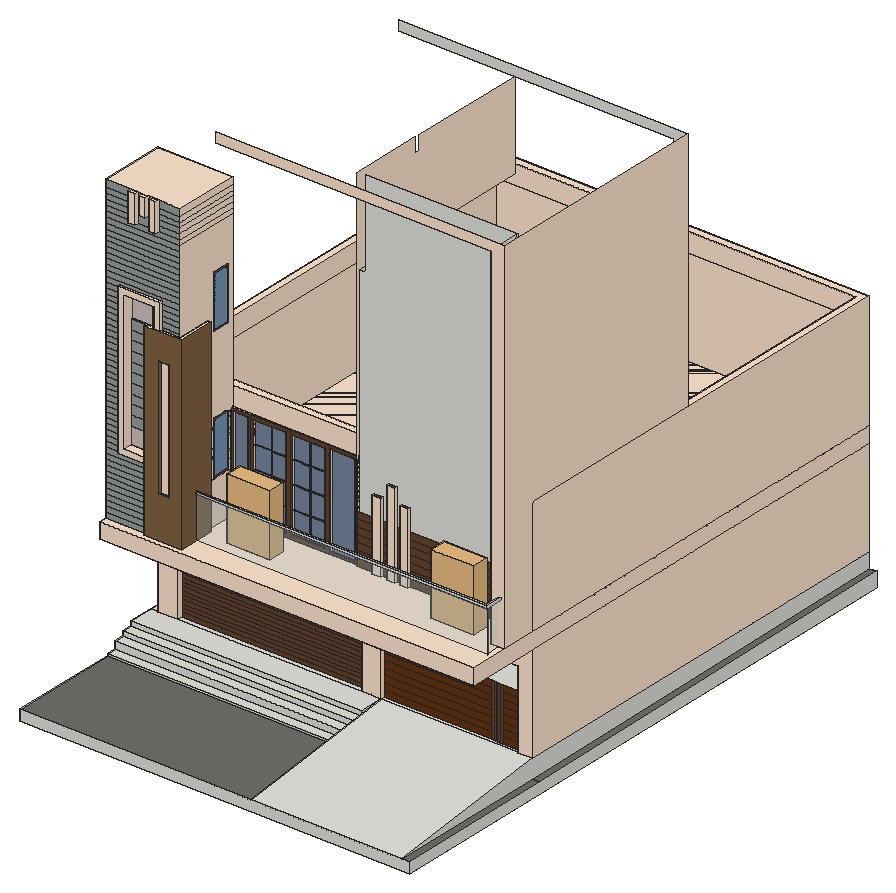
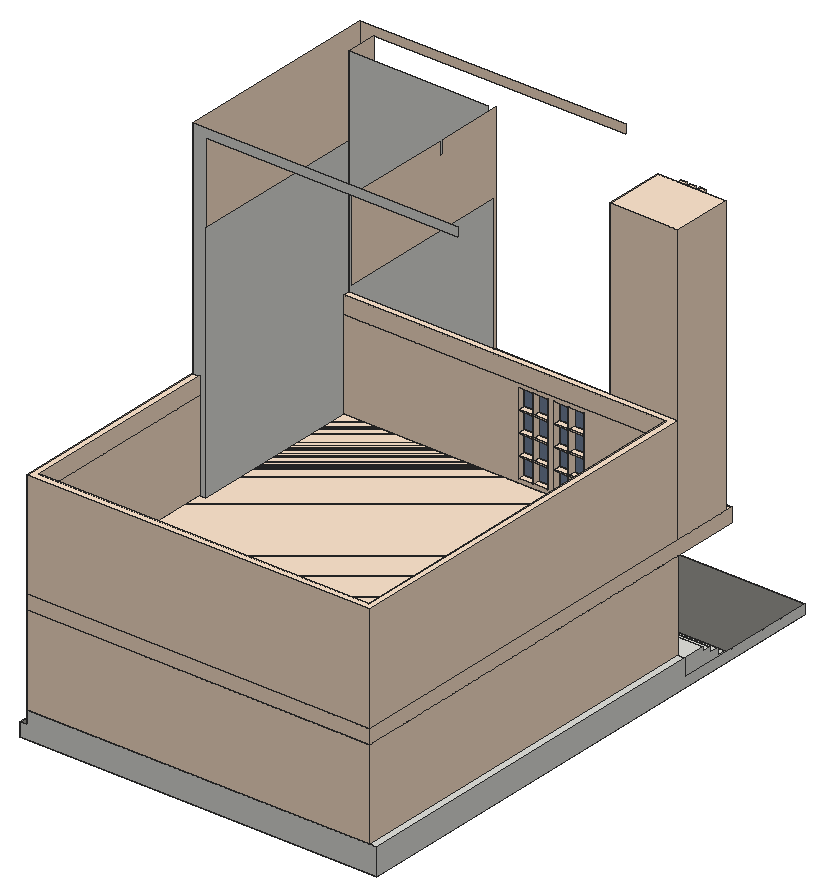
# SketchUp Ruby script. Lengths in inches.
U = 1.inch
M = Sketchup.active_model
def pt(a) = Geom::Point3d.new(a.map { |v| v * U })
def face(e, loops, mat)
  f = e.add_face(loops[0].map { |a| pt(a) })
  loops[1..].each { |l| e.add_face(l.map { |a| pt(a) }).erase! }
  f.material = f.back_material = mat if mat
  f
end
# faces: each face lists its corners as indices into pts; further lists are holes
def faces(e, pts, list, mat = nil) = list.each { |f| face(e, (f[0].is_a?(Array) ? f : [f]).map { |l| l.map { |i| pts[i] } }, mat) }
# xy, xz, yz: faces in a plane at the given z, y or x. An outline is a flat list of corners, or four numbers for a rectangle; further outlines are holes
def ring(l) = l.size == 4 ? [[l[0], l[1]], [l[2], l[1]], [l[2], l[3]], [l[0], l[3]]] : l.each_slice(2).to_a
def flat(e, list, mat, &to3) = list.each { |f| face(e, (f[0].is_a?(Array) ? f : [f]).map { |l| ring(l).map { |u, v| to3.(u, v) } }, mat) }
def xy(e, z, list, mat = nil) = flat(e, list, mat) { |x, y| [x, y, z] }
def xz(e, y, list, mat = nil) = flat(e, list, mat) { |x, z| [x, y, z] }
def yz(e, x, list, mat = nil) = flat(e, list, mat) { |y, z| [x, y, z] }
def lines(e, pts, list) = list.each { |a, b| e.add_line(pt(pts[a]), pt(pts[b])) }
# prism: a flat outline (further loops are holes) pulled along v
def prism(e, loops, v, mat = nil)
  f = face(e, loops, mat); d = Geom::Vector3d.new(v.map { |x| x * U })
  f.pushpull(f.normal.samedirection?(d) ? d.length : -d.length)
end
def box(e, o, s, mat = nil) = prism(e, [[o, [o[0] + s[0], o[1], o[2]], [o[0] + s[0], o[1] + s[1], o[2]], [o[0], o[1] + s[1], o[2]]]], [0, 0, s[2]], mat)
def at(x, y, z, deg = 0) = Geom::Transformation.translation(pt([x, y, z])) * Geom::Transformation.rotation(ORIGIN, Z_AXIS, deg.degrees)
def axes(o, x, y, z) = Geom::Transformation.new([*x, 0, *y, 0, *z, 0, *pt(o).to_a, 1])
def part(name) = M.definitions.add(name)
# library, detail: a bought-in or finely detailed component or shape, given as its bounding box
def library(name, o, s) = part(name).tap { |d| box(d.entities, o, s) }
def detail(e, o, s) = box(e.add_group.entities, o, s)
def put(e, d, t, mat = nil) = e.add_instance(d, t).tap { |i| i.material = mat if mat }
def group(e, t, mat = nil) = e.add_group.tap { |g| g.transformation = t; g.material = mat if mat }.entities
root = M.entities
M.materials.add("C01_Vanilla_Cream").color = [255, 230, 206]
M.materials.add("Glass_Mirror_01").color = [119, 135, 160]
M.materials.add("Glass_Mirror_2").color = [118, 153, 185]
M.materials.add("Glass_Safety_1").color = [204, 235, 244]
M.materials["Glass_Safety_1"].alpha = 0.25
M.materials.add("Glass_Sky Reflection_01").color = [126, 138, 183]
M.materials["Glass_Sky Reflection_01"].alpha = 0.25
M.materials.add("M03_Pewter_Shine").color = [152, 160, 157]
M.materials.add("Plywood_01_1K").color = [104, 52, 18]
M.materials.add("Plywood_01_1K1").color = [130, 99, 66]
M.materials.add("Plywood_01_1K2").color = [125, 96, 64]
M.materials.add("Tile_Exterior_07_1K").color = [112, 111, 107]
M.materials.add("Wood_Veneer_15_1K").color = [103, 69, 45]
c1 = library("Group_2",[-1.28,-0.39,0],[21.22,20.51,48.44])
xy(root,139,[[465.23,139.58,463.25,158.82,463.38,158.82,465.57,139.58],[453,158.82,453,441,471,441,471,158.82,463.38,158.82,462,170.99,462,158.82],[462,158.82,462,170.99,463.25,158.82],[463.25,158.82,462,170.99,463.38,158.82],[278.18,194.51,288.54,198],
  [256.9,198,453,201]])
xy(root,191.09,[[105.48,138.27,465.23,139.58],[105.48,139.58,105.48,141.07,462.4,141.07,462.4,165.41,462.58,165.41,465.23,139.58],[465.23,139.58,462.58,165.41,465.23,165.41]])
xz(root,138.27,[[105.48,191.09,465.23,193.67]])
xz(root,139.58,[[465.23,139,465.57,191.09],[105.48,191.09,465.57,191.09,462,191.2,105.48,191.2]])
xz(root,139.58,[[105.48,139,465.23,191.09]],"Glass_Safety_1")
xz(root,141.07,[[105.48,191.09,462.4,193.67]])
xz(root,158.82,[[453,139,471,139,471,585,114,585,114,573,453,573]],"C01_Vanilla_Cream")
xz(root,165.41,[[462.4,191.09,465.23,193.67]])
xz(root,194.51,[[278.18,139,288.54,225.8],[296.18,139,306.54,243.16],[312.12,139,322.48,225.8]],"C01_Vanilla_Cream")
xz(root,198,[[256.9,139,278.18,147.68],[278.18,139,288.54,147.68],[288.54,139,296.18,147.68],[296.18,139,306.54,147.68],[306.54,139,312.12,147.68],
  [312.12,139,322.48,147.68],[322.48,139,453,147.68],[256.9,147.68,278.18,156.36],[278.18,147.68,288.54,225.8],[288.54,147.68,296.18,156.36],
  [296.18,147.68,306.54,243.16],[306.54,147.68,312.12,156.36],[312.12,147.68,322.48,225.8],[322.48,147.68,453,156.36],[256.9,156.36,278.18,165.04],
  [288.54,156.36,296.18,165.04],[306.54,156.36,312.12,165.04],[322.48,156.36,453,165.04],[256.9,165.04,278.18,173.72],[288.54,165.04,296.18,173.72],
  [306.54,165.04,312.12,173.72],[322.48,165.04,453,173.72],[256.9,173.72,278.18,182.4],[288.54,173.72,296.18,182.4],[306.54,173.72,312.12,182.4],
  [322.48,173.72,453,182.4],[256.9,182.4,278.18,191.08],[288.54,182.4,296.18,191.08],[306.54,182.4,312.12,191.08],[322.48,182.4,453,191.08],
  [256.9,191.08,278.18,199.76],[288.54,191.08,296.18,199.76],[306.54,191.08,312.12,199.76],[322.48,191.08,453,199.76]],"Wood_Veneer_15_1K")
xz(root,201,[[256.9,139,256.9,465,265.5,465,265.5,573,453,573,453,139]])
xz(root,205.5,[[284.33,0,416.71,8.16],[430.63,0,453,8.16],[284.33,8.16,416.71,16.33],[430.63,8.16,453,16.33],[284.33,16.33,416.71,24.49],
  [430.63,16.33,453,24.49],[284.33,24.49,416.71,32.65],[430.63,24.49,453,32.65],[284.33,32.65,416.71,40.82],[430.63,32.65,453,40.82],
  [284.33,40.82,416.71,48.98],[430.63,40.82,453,48.98],[284.33,48.98,416.71,57.14],[430.63,48.98,453,57.14],[284.33,57.14,416.71,65.31],
  [430.63,57.14,453,65.31]],"Plywood_01_1K")
xz(root,205.5,[[416.71,0,419.71,65.31],[419.71,0,422.27,65.31],[422.27,0,425.27,65.31],[425.27,0,427.63,65.31],[427.63,0,430.63,65.31]],"Wood_Veneer_15_1K")
xz(root,441,[[453,139,453,573,114,573,114,585,471,585,471,139]])
yz(root,105.48,[[138.27,191.09,141.07,193.67]])
yz(root,256.9,[[198,139,198,573,287.91,573,287.91,555.9375,293.09,555.9375,293.09,573,441,573,441,465,201,465,201,139]],"C01_Vanilla_Cream")
yz(root,278.18,[[194.51,139,198,225.8]],"C01_Vanilla_Cream")
yz(root,288.54,[[194.51,139,198,225.8]],"C01_Vanilla_Cream")
yz(root,296.18,[[194.51,139,198,243.16]],"C01_Vanilla_Cream")
yz(root,306.54,[[194.51,139,198,243.16]],"C01_Vanilla_Cream")
yz(root,312.12,[[194.51,139,198,225.8]])
yz(root,322.48,[[194.51,139,198,225.8]],"C01_Vanilla_Cream")
yz(root,453,[[198,139,201,573],[201,139,441,465]])
yz(root,453,[[158.82,139,198,573]],"C01_Vanilla_Cream")
yz(root,462.4,[[141.07,191.09,165.41,193.67]])
yz(root,465.23,[[138.27,191.09,165.41,193.67]])
yz(root,471,[[158.82,139,441,585]],"C01_Vanilla_Cream")
p = [[465.23,139.58,191.09],[462.58,165.41,191.09],[462,170.99,191.09],[462,170.99,139],[463.25,158.82,139],[465.23,139.58,139],
  [105.48,139.58,191.2],[105.48,139.58,193],[2323.11,2299.07,-227.3],[2323.11,2299.07,-224.27],[2323.11,2299.07,-230.33],[2331.43,2299.07,-221.25],
  [2331.45,2299.07,-233.35],[2331.43,2299.07,-233.35],[2331.45,2299.07,-221.25]]
faces(root,p,[[0,1,2,3,4,5]],"Glass_Safety_1")
lines(root,p,[[6,7],[8,9],[10,8],[9,11],[12,13],[11,14],[13,10]])
g1 = group(root,at(0,0,-36))
xy(g1,0,[[0,0,480,720]])
xy(g1,12.99,[[284.33,0,471,201]])
xy(g1,12.99,[[0,0,284.33,134.43],[471,0,480,201]],"Tile_Exterior_07_1K")
xy(g1,15.375,[[0,134.43,284.33,146.43]])
xy(g1,24.09,[[0,146.43,284.33,158.43]])
xy(g1,30.22,[[0,158.43,284.33,170.43]])
xy(g1,36,[[0,170.43,284.33,201],[0,201,471,720]])
xz(g1,0,[[0,0,480,12.99]])
xz(g1,134.43,[[0,12.99,284.33,15.375]])
xz(g1,146.43,[[0,15.375,284.33,24.09]])
xz(g1,158.43,[[0,24.09,284.33,30.22]])
xz(g1,170.43,[[0,30.22,284.33,36]])
xz(g1,720,[[0,0,0,36,471,36,471,18,480,18,480,0]])
yz(g1,0,[[0,0,0,12.99,201,12.99,201,36,720,36,720,0],[134.43,12.99,134.43,15.375,146.43,15.375,146.43,24.09,158.43,24.09,158.43,30.22,170.43,30.22,170.43,36,201,36,201,12.99]])
yz(g1,284.33,[[0,12.99,170.43,32.5,170.43,30.22,158.43,30.22,158.43,24.09,146.43,24.09,146.43,15.375,134.43,15.375,134.43,12.99],[134.43,12.99,201,12.99,201,36,170.43,32.5,170.43,30.22,158.43,30.22,158.43,24.09,146.43,24.09,146.43,15.375,134.43,15.375],[170.43,32.5,201,36,170.43,36]])
yz(g1,471,[[0,12.99,201,12.99,720,18,720,36,201,36]])
yz(g1,480,[[0,0,720,0,720,18,201,12.99,0,12.99]])
p = [[284.33,201,36],[284.33,170.43,32.5],[284.33,0,12.99],[457.43,0,12.99],[471,0,12.99],[471,201,36],
  [480,201,12.99],[480,720,18],[471,720,18],[471,201,12.99]]
faces(g1,p,[[0,1,2,3,4,5]])
faces(g1,p,[[6,7,8,9]],"Tile_Exterior_07_1K")
g2 = group(root,at(9,201,0),"C01_Vanilla_Cream")
xy(g2,0,[[[0,0,24,0,24,6.24,251.33,6.24,251.33,0,263.33,0,275.33,9,275.33,188.59,453,188.59,453,9,444,9,444,0,462,0,462,519,0,519],[9,9,9,510,453,510,453,200.35,263.33,200.35,263.33,9]],[263.33,0,275.33,0,275.33,9],[9,9,263.33,9,263.33,200.35,453,200.35,453,510,9,510],[275.33,9,453,188.59]])
xy(g2,7.84,[[327.57,194.47,371.57,200.35]])
xy(g2,7.84,[[327.57,188.59,371.57,194.47]],"Wood_Veneer_15_1K")
xy(g2,96,[[24,0,251.33,6.24],[275.33,0,444,9]])
xy(g2,100.92,[[327.57,194.47,371.57,200.35]])
xy(g2,100.92,[[327.57,188.59,371.57,194.47]],"Wood_Veneer_15_1K")
xy(g2,120,[[[0,0,462,519],[9,9,9,510,453,510,453,200.35,263.33,200.35,263.33,9],[275.33,9,453,188.59]]])
xz(g2,0,[[0,0,24,0,24,96,251.33,96,251.33,0,275.33,0,275.33,96,444,96,444,0,462,0,462,120,0,120]])
xz(g2,6.24,[[24,0,251.33,4.8],[24,4.8,251.33,9.6],[24,9.6,251.33,14.4],[24,14.4,251.33,19.2],[24,19.2,251.33,24],
  [24,24,251.33,28.8],[24,28.8,251.33,33.6],[24,33.6,251.33,38.4],[24,38.4,251.33,43.2],[24,43.2,251.33,48],
  [24,48,251.33,52.8],[24,52.8,251.33,57.6],[24,57.6,251.33,62.4],[24,62.4,251.33,67.2],[24,67.2,251.33,72],
  [24,72,251.33,76.8],[24,76.8,251.33,81.6],[24,81.6,251.33,86.4],[24,86.4,251.33,91.2],[24,91.2,251.33,96]],"Wood_Veneer_15_1K")
xz(g2,9,[[9,0,263.33,120],[444,0,444,96,275.33,96,275.33,120,453,120,453,0]])
xz(g2,188.59,[[[275.33,0,453,120],[327.57,7.84,371.57,100.92]]],"Plywood_01_1K2")
xz(g2,194.47,[[327.57,7.84,371.57,100.92]],"Wood_Veneer_15_1K")
xz(g2,200.35,[[[263.33,0,453,120],[327.57,7.84,371.57,100.92]]])
xz(g2,510,[[9,0,453,120]])
xz(g2,519,[[0,0,462,120]])
yz(g2,0,[[0,0,519,120]])
yz(g2,9,[[9,0,510,120]])
yz(g2,24,[[0,0,6.24,96]])
yz(g2,251.33,[[0,0,6.24,96]])
yz(g2,263.33,[[9,0,200.35,120]])
yz(g2,275.33,[[0,0,188.59,0,188.59,120,9,120,9,96,0,96]])
yz(g2,327.57,[[194.47,7.84,200.35,100.92]])
yz(g2,327.57,[[188.59,7.84,194.47,100.92]],"Wood_Veneer_15_1K")
yz(g2,371.57,[[194.47,7.84,200.35,100.92]])
yz(g2,371.57,[[188.59,7.84,194.47,100.92]],"Wood_Veneer_15_1K")
yz(g2,444,[[0,0,9,96]])
yz(g2,453,[[9,0,188.59,120],[188.59,0,200.35,120],[200.35,0,510,120]])
yz(g2,462,[[0,0,519,120]])
p = [[263.33,0,0],[263.33,9,120]]
lines(g2,p,[[0,1]])
g3 = group(root,at(9,201,120),"C01_Vanilla_Cream")
xy(g3,0,[[0,-89.98,462,519]])
xy(g3,19,[[0,-89.98,462,-89.98,462,519,0,519,0,0,91.9,0,91.9,-38.7,96.48,-38.7,96.48,-84.13,50.47,-84.13,50.47,-80.45,0,-80.45],[0,-80.45,91.9,0]])
xy(g3,71.29,[[68.81,-84.13,81.2,-81.02]],"Plywood_01_1K1")
xy(g3,97.51,[[17.03,-83.45,50.47,-80.45]])
xy(g3,104.51,[[24.03,-83.45,50.47,-83.45,50.47,-80.45,61.96,-80.45,61.96,-71.76,24.03,-71.76]])
xy(g3,217.73,[[68.81,-84.13,81.2,-81.02]],"Plywood_01_1K1")
xy(g3,243.18,[[24.03,-71.76,50.48,-69.76]])
xy(g3,250.46,[[50.47,-84.13,96.48,-84.13,96.48,-38.7,91.9,-38.7,91.9,-80.45,50.47,-80.45]])
xy(g3,250.6,[[61.96,-83.45,68.96,-80.45]])
xy(g3,275.37,[[24.03,-83.45,24.03,-69.76,50.48,-69.76,50.48,-71.76,61.96,-71.76,61.96,-83.45]])
xy(g3,282.37,[[17.03,-83.45,68.96,-80.45]])
xy(g3,358.04,[[31.4,-85.45,39.37,-80.45],[57.05,-85.45,65.02,-80.45]])
xy(g3,371.08,[[44.54,-85.45,52.51,-80.45]])
xy(g3,393,[[31.4,-85.45,39.37,-80.45],[44.54,-85.45,52.51,-80.45],[57.05,-85.45,65.02,-80.45],[0,-80.45,91.9,0]])
xz(g3,-89.98,[[0,0,462,19]])
xz(g3,-85.45,[[31.4,358.04,39.37,393],[57.05,358.04,65.02,393],[44.54,371.08,52.51,393]])
xz(g3,-84.13,[[[50.47,19,96.48,250.46],[68.81,71.29,81.2,217.73]]],"Plywood_01_1K1")
xz(g3,-83.45,[[17.03,97.51,50.47,97.51,50.47,104.51,24.03,104.51,24.03,275.37,61.96,275.37,61.96,250.6,68.96,250.6,68.96,282.37,17.03,282.37]])
xz(g3,-81.02,[[68.81,71.29,81.2,217.73]])
xz(g3,-80.45,[[50.47,19,91.9,25.52],[50.47,25.52,91.9,32.04],[50.47,32.04,91.9,38.56],[50.47,38.56,91.9,45.08],[50.47,45.08,91.9,51.6],
  [50.47,51.6,91.9,58.12],[50.47,58.12,91.9,64.64],[50.47,64.64,91.9,64.64,91.9,247.2,68.96,247.2,68.96,250.46,61.96,250.46,61.96,104.51,50.47,104.51],[50.47,104.51,61.96,250.46],[61.96,250.46,68.96,250.6],
  [31.4,358.04,39.37,393],[57.05,358.04,65.02,393],[44.54,371.08,52.51,393]])
xz(g3,-80.45,[[0,19,50.47,25.52],[0,25.52,50.47,32.04],[0,32.04,50.47,38.56],[0,38.56,50.47,45.08],[0,45.08,50.47,51.6],
  [0,51.6,50.47,58.12],[0,58.12,50.47,64.64],[0,64.64,50.47,71.16],[0,71.16,50.47,77.68],[0,77.68,50.47,84.2],
  [0,84.2,50.47,90.72],[0,90.72,50.47,97.24],[0,97.24,50.47,97.24,50.47,97.51,17.03,97.51,17.03,103.76,0,103.76],[0,103.76,17.03,110.28],[0,110.28,17.03,116.8],
  [0,116.8,17.03,123.32],[0,123.32,17.03,129.84],[0,129.84,17.03,136.36],[0,136.36,17.03,142.88],[0,142.88,17.03,149.4],
  [0,149.4,17.03,155.92],[0,155.92,17.03,162.44],[0,162.44,17.03,168.96],[0,168.96,17.03,175.48],[0,175.48,17.03,182],
  [0,182,17.03,188.52],[0,188.52,17.03,195.04],[0,195.04,17.03,201.56],[0,201.56,17.03,208.08],[0,208.08,17.03,214.6],
  [0,214.6,17.03,221.12],[0,221.12,17.03,227.64],[0,227.64,17.03,234.16],[0,234.16,17.03,240.68],[0,240.68,17.03,247.2],
  [0,247.2,17.03,253.72],[68.96,247.2,91.9,250.46],[68.96,250.46,91.9,253.72],[0,253.72,17.03,260.24],[68.96,253.72,91.9,260.24],
  [0,260.24,17.03,266.76],[68.96,260.24,91.9,266.76],[0,266.76,17.03,273.28],[68.96,266.76,91.9,273.28],[0,273.28,17.03,279.8],
  [68.96,273.28,91.9,279.8],[0,279.8,17.03,279.8,17.03,282.37,68.96,282.37,68.96,279.8,91.9,279.8,91.9,286.32,0,286.32],[0,286.32,91.9,292.84],[0,292.84,91.9,299.36],[0,299.36,91.9,305.88],
  [0,305.88,91.9,312.4],[0,312.4,91.9,318.92],[0,318.92,91.9,325.44],[0,325.44,91.9,331.96],[0,331.96,91.9,338.48],
  [0,338.48,91.9,345],[0,345,91.9,351.52],[0,351.52,91.9,358.04],[0,358.04,31.4,364.56],[39.37,358.04,57.05,358.04,57.05,393,52.51,393,52.51,371.08,44.54,371.08,44.54,393,39.37,393],
  [65.02,358.04,91.9,364.56],[0,364.56,31.4,371.08],[65.02,364.56,91.9,371.08],[0,371.08,31.4,377.6],[65.02,371.08,91.9,377.6],
  [0,377.6,31.4,384.12],[65.02,377.6,91.9,384.12],[0,384.12,31.4,393],[65.02,384.12,91.9,393]],"M03_Pewter_Shine")
xz(g3,-71.76,[[24.03,104.51,61.96,125.46]],"Glass_Sky Reflection_01")
xz(g3,-71.76,[[24.03,125.46,61.96,137.23],[24.03,137.23,61.96,149.01],[24.03,149.01,61.96,160.78],[24.03,160.78,61.96,172.55],[24.03,172.55,61.96,184.32],
  [24.03,184.32,61.96,196.09],[24.03,196.09,61.96,207.87],[24.03,207.87,61.96,219.64],[24.03,219.64,61.96,231.41],[24.03,231.41,61.96,243.18],
  [50.48,243.18,61.96,249.62],[50.48,249.62,61.96,256.06],[50.48,256.06,61.96,262.5],[50.48,262.5,61.96,268.93],[50.48,268.93,61.96,275.37]],"M03_Pewter_Shine")
xz(g3,-69.76,[[24.03,243.18,50.48,275.37]],"Glass_Sky Reflection_01")
xz(g3,-38.7,[[91.9,19,96.48,250.46]])
xz(g3,0,[[0,19,91.9,393]])
xz(g3,519,[[0,0,462,19]])
yz(g3,0,[[-89.98,0,519,19],[-80.45,19,0,393]])
yz(g3,17.03,[[-83.45,97.51,-80.45,282.37]])
yz(g3,24.03,[[-83.45,104.51,-71.76,104.51,-71.76,243.18,-69.76,243.18,-69.76,275.37,-83.45,275.37]])
yz(g3,31.4,[[-85.45,358.04,-80.45,393]])
yz(g3,39.37,[[-85.45,358.04,-80.45,393]])
yz(g3,44.54,[[-85.45,371.08,-80.45,393]])
yz(g3,50.47,[[-84.13,19,-84.13,250.46,-83.45,250.46,-83.45,97.51,-80.45,97.51,-80.45,19],[-83.45,97.51,-80.45,104.51],[-83.45,104.51,-80.45,250.46]])
yz(g3,50.48,[[-71.76,243.18,-69.76,249.62],[-71.76,249.62,-69.76,256.06],[-71.76,256.06,-69.76,262.5],[-71.76,262.5,-69.76,268.93],[-71.76,268.93,-69.76,275.37]])
yz(g3,52.51,[[-85.45,371.08,-80.45,393]])
yz(g3,57.05,[[-85.45,358.04,-80.45,393]])
yz(g3,61.96,[[-80.45,104.51,-80.45,250.6,-83.45,250.6,-83.45,275.37,-71.76,275.37,-71.76,104.51]])
yz(g3,65.02,[[-85.45,358.04,-80.45,393]])
yz(g3,68.81,[[-84.13,71.29,-81.02,217.73]],"Plywood_01_1K1")
yz(g3,68.96,[[-83.45,250.6,-80.45,282.37]])
yz(g3,81.2,[[-84.13,71.29,-81.02,217.73]],"Plywood_01_1K1")
yz(g3,91.9,[[-80.45,19,-38.7,250.46],[[-38.7,19,0,19,0,351.52,-80.45,351.52,-80.45,250.46,-38.7,250.46],[-30.47,71.51,-5.73,139.15],[-30.47,233.3,-5.73,300.9375]],[-80.45,351.52,0,358.04],[-80.45,358.04,0,364.56],[-80.45,364.56,0,371.08],
  [-80.45,371.08,0,377.6],[-80.45,377.6,0,384.12],[-80.45,384.12,0,393]])
yz(g3,91.9,[[-27.47,74.51,-8.73,136.15],[-27.47,236.3,-8.73,297.9375]],"Glass_Mirror_2")
yz(g3,91.9,[[[-30.47,71.51,-5.73,139.15],[-27.47,74.51,-8.73,136.15]],[[-30.47,233.3,-5.73,300.9375],[-27.47,236.3,-8.73,297.9375]]],"Wood_Veneer_15_1K")
yz(g3,96.48,[[-84.13,19,-38.7,250.46]],"Plywood_01_1K1")
yz(g3,462,[[-89.98,0,519,19]])
p = [[17.03,-80.45,279.8],[68.96,-80.45,279.8],[17.03,-80.45,103.76],[50.47,-80.45,103.76]]
lines(g3,p,[[0,1],[2,3]])
put(root,c1,axes([134.18,155.33,139],[2.485,0,0],[0,1,0],[0,0,1.57]))
put(root,c1,axes([380.18,162.13,139],[2.485,0,0],[0,1,0],[0,0,1.57]))
g4 = group(root,at(9,201,139),"C01_Vanilla_Cream")
xy(g4,0,[[[91.9,-2,247.9,-2,247.9,0,462,0,462,519,0,519,0,0,91.9,0],[9,9,453,510]],[9,9,453,510]])
xy(g4,3,[[94.9,-2,112.9,0],[214.9,-2,244.9,0]])
xy(g4,4,[[119.9,-2,139.9,0],[139.9,-2,140.9,0],[140.9,-2,159.9,0],[167.9,-2,187.9,0],[187.9,-2,188.9,0],
  [188.9,-2,207.9,0]])
xy(g4,5,[[119.9,0,139.9,9],[140.9,0,159.9,9],[167.9,0,187.9,9],[188.9,0,207.9,9]])
xy(g4,31.75,[[119.9,0,139.9,9],[140.9,0,159.9,9],[167.9,0,187.9,9],[188.9,0,207.9,9]])
xy(g4,32.75,[[119.9,0,139.9,9],[140.9,0,159.9,9],[167.9,0,187.9,9],[188.9,0,207.9,9]])
xy(g4,59.5,[[119.9,0,139.9,9],[140.9,0,159.9,9],[167.9,0,187.9,9],[188.9,0,207.9,9]])
xy(g4,60.5,[[119.9,0,139.9,9],[140.9,0,159.9,9],[167.9,0,187.9,9],[188.9,0,207.9,9]])
xy(g4,87.25,[[119.9,0,139.9,9],[140.9,0,159.9,9],[167.9,0,187.9,9],[188.9,0,207.9,9]])
xy(g4,88.25,[[119.9,0,139.9,9],[140.9,0,159.9,9],[167.9,0,187.9,9],[188.9,0,207.9,9]])
xy(g4,115,[[119.9,0,139.9,9],[140.9,0,159.9,9],[167.9,0,187.9,9],[188.9,0,207.9,9]])
xy(g4,116,[[119.9,-2,139.9,0],[139.9,-2,140.9,0],[140.9,-2,159.9,0],[167.9,-2,187.9,0],[187.9,-2,188.9,0],
  [188.9,-2,207.9,0]])
xy(g4,117,[[94.9,-2,112.9,0],[214.9,-2,244.9,0]])
xy(g4,120,[[91.9,-2,115.9,0],[115.9,-2,163.9,0],[163.9,-2,211.9,0],[211.9,-2,247.9,0]])
xy(g4,144,[[[0,0,462,519],[9,9,453,510]]])
xz(g4,-2,[[[91.9,0,115.9,120],[94.9,3,112.9,117]],[[115.9,0,163.9,120],[119.9,4,159.9,116]],[[163.9,0,211.9,120],[167.9,4,207.9,116]],[[211.9,0,247.9,120],[214.9,3,244.9,117]]],"Wood_Veneer_15_1K")
xz(g4,0,[[0,0,91.9,0,91.9,120,247.9,120,247.9,144,0,144],[247.9,0,462,120],[119.9,4,139.9,5],[139.9,4,140.9,5],[140.9,4,159.9,5],
  [167.9,4,187.9,5],[187.9,4,188.9,5],[188.9,4,207.9,5],[139.9,5,140.9,31.75],[187.9,5,188.9,31.75],
  [119.9,31.75,139.9,32.75],[139.9,31.75,140.9,32.75],[140.9,31.75,159.9,32.75],[167.9,31.75,187.9,32.75],[187.9,31.75,188.9,32.75],
  [188.9,31.75,207.9,32.75],[139.9,32.75,140.9,59.5],[187.9,32.75,188.9,59.5],[119.9,59.5,139.9,60.5],[139.9,59.5,140.9,60.5],
  [140.9,59.5,159.9,60.5],[167.9,59.5,187.9,60.5],[187.9,59.5,188.9,60.5],[188.9,59.5,207.9,60.5],[139.9,60.5,140.9,87.25],
  [187.9,60.5,188.9,87.25],[119.9,87.25,139.9,88.25],[139.9,87.25,140.9,88.25],[140.9,87.25,159.9,88.25],[167.9,87.25,187.9,88.25],
  [187.9,87.25,188.9,88.25],[188.9,87.25,207.9,88.25],[139.9,88.25,140.9,115],[187.9,88.25,188.9,115],[119.9,115,139.9,116],
  [139.9,115,140.9,116],[140.9,115,159.9,116],[167.9,115,187.9,116],[187.9,115,188.9,116],[188.9,115,207.9,116],
  [247.9,120,462,144]])
xz(g4,0,[[94.9,3,112.9,117],[214.9,3,244.9,117],[119.9,5,139.9,31.75],[140.9,5,159.9,31.75],[167.9,5,187.9,31.75],
  [188.9,5,207.9,31.75],[119.9,32.75,139.9,59.5],[140.9,32.75,159.9,59.5],[167.9,32.75,187.9,59.5],[188.9,32.75,207.9,59.5],
  [119.9,60.5,139.9,87.25],[140.9,60.5,159.9,87.25],[167.9,60.5,187.9,87.25],[188.9,60.5,207.9,87.25],[119.9,88.25,139.9,115],
  [140.9,88.25,159.9,115],[167.9,88.25,187.9,115],[188.9,88.25,207.9,115]],"Glass_Mirror_01")
xz(g4,9,[[[9,0,453,120],[119.9,60.5,139.9,87.25],[119.9,88.25,139.9,115],[119.9,32.75,139.9,59.5],[119.9,5,139.9,31.75],[167.9,60.5,187.9,87.25],[167.9,88.25,187.9,115],[167.9,32.75,187.9,59.5],[167.9,5,187.9,31.75],[140.9,88.25,159.9,115],[140.9,32.75,159.9,59.5],[140.9,5,159.9,31.75],[140.9,60.5,159.9,87.25],[188.9,88.25,207.9,115],[188.9,60.5,207.9,87.25],[188.9,32.75,207.9,59.5],[188.9,5,207.9,31.75]],[9,120,453,144]])
xz(g4,510,[[9,0,453,120],[9,120,453,144]])
xz(g4,519,[[0,0,462,144]])
yz(g4,0,[[0,0,519,144]])
yz(g4,9,[[9,0,510,120],[9,120,510,144]])
yz(g4,91.9,[[-2,0,0,120]])
yz(g4,94.9,[[-2,3,0,117]])
yz(g4,112.9,[[-2,3,0,117]])
yz(g4,119.9,[[-2,4,0,5],[-2,5,0,31.75],[0,5,9,31.75],[-2,31.75,0,32.75],[-2,32.75,0,59.5],
  [0,32.75,9,59.5],[-2,59.5,0,60.5],[-2,60.5,0,87.25],[0,60.5,9,87.25],[-2,87.25,0,88.25],
  [-2,88.25,0,115],[0,88.25,9,115],[-2,115,0,116]])
yz(g4,139.9,[[0,5,9,31.75],[0,32.75,9,59.5],[0,60.5,9,87.25],[0,88.25,9,115]])
yz(g4,140.9,[[0,5,9,31.75],[0,32.75,9,59.5],[0,60.5,9,87.25],[0,88.25,9,115]])
yz(g4,159.9,[[-2,4,0,5],[-2,5,0,31.75],[0,5,9,31.75],[-2,31.75,0,32.75],[-2,32.75,0,59.5],
  [0,32.75,9,59.5],[-2,59.5,0,60.5],[-2,60.5,0,87.25],[0,60.5,9,87.25],[-2,87.25,0,88.25],
  [-2,88.25,0,115],[0,88.25,9,115],[-2,115,0,116]])
yz(g4,167.9,[[-2,4,0,5],[-2,5,0,31.75],[0,5,9,31.75],[-2,31.75,0,32.75],[-2,32.75,0,59.5],
  [0,32.75,9,59.5],[-2,59.5,0,60.5],[-2,60.5,0,87.25],[0,60.5,9,87.25],[-2,87.25,0,88.25],
  [-2,88.25,0,115],[0,88.25,9,115],[-2,115,0,116]])
yz(g4,187.9,[[0,5,9,31.75],[0,32.75,9,59.5],[0,60.5,9,87.25],[0,88.25,9,115]])
yz(g4,188.9,[[0,5,9,31.75],[0,32.75,9,59.5],[0,60.5,9,87.25],[0,88.25,9,115]])
yz(g4,207.9,[[-2,4,0,5],[-2,5,0,31.75],[0,5,9,31.75],[-2,31.75,0,32.75],[-2,32.75,0,59.5],
  [0,32.75,9,59.5],[-2,59.5,0,60.5],[-2,60.5,0,87.25],[0,60.5,9,87.25],[-2,87.25,0,88.25],
  [-2,88.25,0,115],[0,88.25,9,115],[-2,115,0,116]])
yz(g4,214.9,[[-2,3,0,117]])
yz(g4,244.9,[[-2,3,0,117]])
yz(g4,247.9,[[-2,0,0,120]])
yz(g4,453,[[9,0,510,120],[9,120,510,144]])
yz(g4,462,[[0,0,519,144]])
